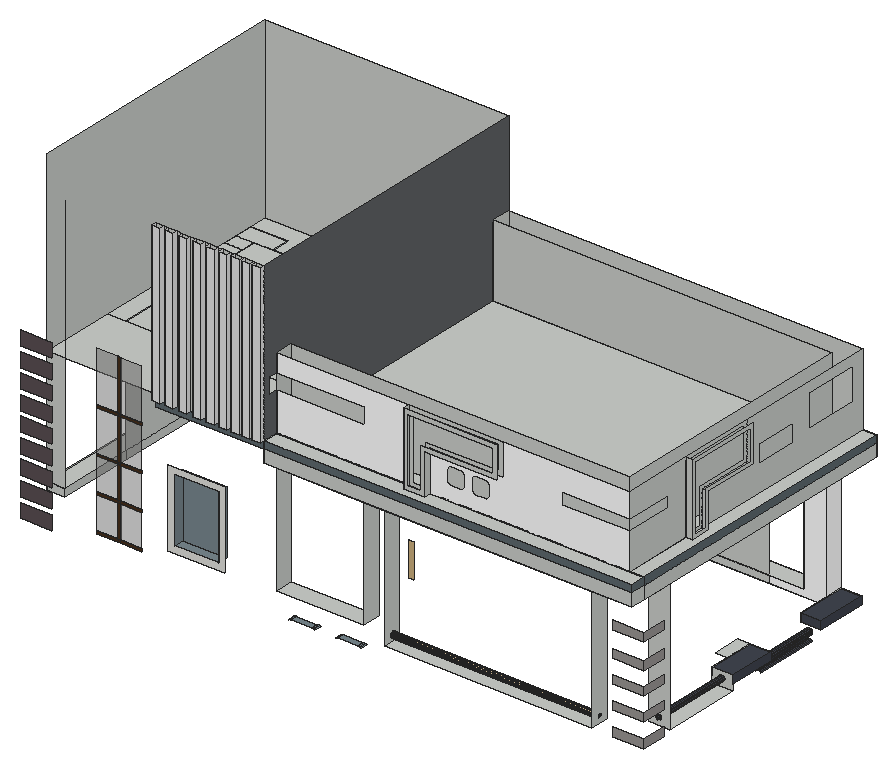
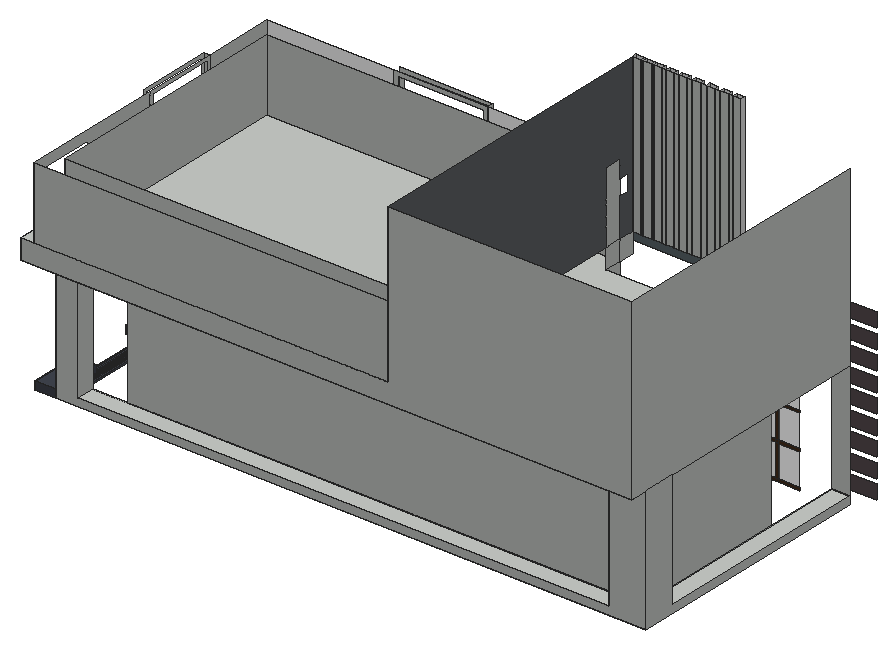
# SketchUp Ruby script. Lengths in inches.
U = 1.inch
M = Sketchup.active_model
def pt(a) = Geom::Point3d.new(a.map { |v| v * U })
def face(e, loops, mat)
  f = e.add_face(loops[0].map { |a| pt(a) })
  loops[1..].each { |l| e.add_face(l.map { |a| pt(a) }).erase! }
  f.material = f.back_material = mat if mat
  f
end
# faces: each face lists its corners as indices into pts; further lists are holes
def faces(e, pts, list, mat = nil) = list.each { |f| face(e, (f[0].is_a?(Array) ? f : [f]).map { |l| l.map { |i| pts[i] } }, mat) }
# xy, xz, yz: faces in a plane at the given z, y or x. An outline is a flat list of corners, or four numbers for a rectangle; further outlines are holes
def ring(l) = l.size == 4 ? [[l[0], l[1]], [l[2], l[1]], [l[2], l[3]], [l[0], l[3]]] : l.each_slice(2).to_a
def flat(e, list, mat, &to3) = list.each { |f| face(e, (f[0].is_a?(Array) ? f : [f]).map { |l| ring(l).map { |u, v| to3.(u, v) } }, mat) }
def xy(e, z, list, mat = nil) = flat(e, list, mat) { |x, y| [x, y, z] }
def xz(e, y, list, mat = nil) = flat(e, list, mat) { |x, z| [x, y, z] }
def yz(e, x, list, mat = nil) = flat(e, list, mat) { |y, z| [x, y, z] }
def lines(e, pts, list) = list.each { |a, b| e.add_line(pt(pts[a]), pt(pts[b])) }
# prism: a flat outline (further loops are holes) pulled along v
def prism(e, loops, v, mat = nil)
  f = face(e, loops, mat); d = Geom::Vector3d.new(v.map { |x| x * U })
  f.pushpull(f.normal.samedirection?(d) ? d.length : -d.length)
end
def box(e, o, s, mat = nil) = prism(e, [[o, [o[0] + s[0], o[1], o[2]], [o[0] + s[0], o[1] + s[1], o[2]], [o[0], o[1] + s[1], o[2]]]], [0, 0, s[2]], mat)
def at(x, y, z, deg = 0) = Geom::Transformation.translation(pt([x, y, z])) * Geom::Transformation.rotation(ORIGIN, Z_AXIS, deg.degrees)
def axes(o, x, y, z) = Geom::Transformation.new([*x, 0, *y, 0, *z, 0, *pt(o).to_a, 1])
def part(name) = M.definitions.add(name)
# library, detail: a bought-in or finely detailed component or shape, given as its bounding box
def library(name, o, s) = part(name).tap { |d| box(d.entities, o, s) }
def detail(e, o, s) = box(e.add_group.entities, o, s)
def put(e, d, t, mat = nil) = e.add_instance(d, t).tap { |i| i.material = mat if mat }
def group(e, t, mat = nil) = e.add_group.tap { |g| g.transformation = t; g.material = mat if mat }.entities
root = M.entities
M.materials.add("[Asphalt New]").color = [89, 79, 82]
M.materials.add("[Basic Tile]").color = [203, 206, 202]
M.materials.add("[Blacktop Old 01]").color = [96, 99, 102]
M.materials.add("[Color M00]").color = [255, 255, 255]
M.materials.add("[Concrete Aggregate Smoke]").color = [154, 150, 148]
M.materials.add("[Formica Beige]").color = [211, 187, 149]
M.materials.add("[Formica Laminate Dark]1").color = [65, 69, 79]
M.materials.add("[Formica Speckled Grey]").color = [120, 135, 142]
M.materials.add("[Formica Speckled Grey]1").color = [94, 105, 111]
M.materials.add("[Polished Concrete Old]").color = [229, 229, 229]
M.materials.add("[Translucent Glass Gray]").color = [128, 128, 128]
M.materials["[Translucent Glass Gray]"].alpha = 0.5
M.materials.add("[Wood Floor Light]").color = [204, 176, 127]
M.materials.add("[Wood Floor]").color = [71, 48, 28]
xy(root,488.49,[[753.6875,719.27,788.57,730.52],[837.19,719.27,870.38,730.52]],"[Formica Speckled Grey]")
xy(root,496.0625,[[909.08,730.52,1278.64,762.76]],"[Basic Tile]")
xy(root,499.9375,[[1333.54,788.47,1370.47,928.88]],"[Basic Tile]")
xy(root,510.75,[[282.77,762.76,282.77,1215.04,1333.54,1215.04,1333.54,1182.79,315.01,1182.79,315.01,762.76],[1333.54,1125.19,1370.47,1215.04]],"[Basic Tile]")
xy(root,517.3125,[[716.67,730.52,872.91,762.76]],"[Basic Tile]")
xy(root,524.8125,[[282.77,762.76,315.01,1157.24],[1311.73,963.8,1333.54,1012.73],[348.88,1182.79,1294.14,1215.04]],"[Basic Tile]")
xy(root,524.8125,[[1333.54,928.88,1370.47,1012.73],[1333.54,1125.19,1370.47,1215.04]],"[Formica Laminate Dark]1")
xy(root,544.32,[[557.73,703.09,635.17,720.91]],"[Formica Speckled Grey]")
xy(root,658.7,[[557.73,703.09,635.17,720.91]],"[Formica Speckled Grey]")
xy(root,732.375,[[716.67,703.09,872.91,730.52],[872.91,703.09,909.08,730.52],[909.08,703.09,1278.64,730.52],[1278.64,703.09,1370.47,730.52],[716.67,730.52,716.67,762.76,282.77,762.76,282.77,898.23,1370.47,898.23,1370.47,788.47,1333.54,788.47,1333.54,762.76,1278.64,762.76,1278.64,730.52,909.08,730.52,909.08,762.76,872.91,762.76,872.91,730.52],
  [872.91,730.52,909.08,762.76],[1278.64,730.52,1370.47,762.76],[1333.54,762.76,1370.47,788.47],[282.77,898.23,315.01,1157.24],[315.01,898.23,1230.77,1182.79],
  [1230.77,898.23,1230.77,1247.67,1294.14,1247.67,1294.14,1182.79,1370.47,1182.79,1370.47,898.23],[282.77,1157.24,315.01,1182.79],[282.77,1182.79,348.88,1215.04],[348.88,1182.79,348.88,1215.04,282.77,1215.04,282.77,1247.67,1230.77,1247.67,1230.77,1182.79],[1294.14,1182.79,1333.54,1215.04],
  [1333.54,1182.79,1370.47,1215.04],[1294.14,1215.04,1370.47,1247.67]],"[Basic Tile]")
xy(root,767.875,[[523.06,695.28,537.89,703.09],[545.87,695.28,560.71,703.09],[570.43,695.28,585.27,703.09],[595.93,695.28,610.77,703.09],[619.62,695.28,634.46,703.09],
  [642.37,695.28,657.21,703.09],[664.18,695.28,679.02,703.09],[683.01,695.28,697.85,703.09],[701.84,695.28,716.67,703.09],[716.67,703.09,1370.47,703.09,1370.47,730.52,989.93,730.52,989.93,718.33,952.31,718.33,952.31,730.52,716.67,730.52],
  [952.31,718.33,989.93,730.52],[716.67,730.52,716.67,762.76,1319.77,762.76,1319.77,1212.51,1345.67,1212.51,1345.67,730.52],[1345.67,730.52,1370.47,730.52,1370.47,1247.67,1345.67,1247.67,1345.67,891.02,1356.61,891.02,1356.61,855.93,1345.67,855.93],[716.67,762.76,1319.77,1212.51],[1345.67,855.93,1356.61,891.02],
  [716.67,1212.51,1345.67,1247.67]],"[Basic Tile]")
xz(root,695.28,[[523.06,767.875,537.89,1047.125],[545.87,767.875,560.71,1047.125],[570.43,767.875,585.27,1047.125],[595.93,767.875,610.77,1047.125],[619.62,767.875,634.46,1047.125],
  [642.37,767.875,657.21,1047.125],[664.18,767.875,679.02,1047.125],[683.01,767.875,697.85,1047.125],[701.84,767.875,716.67,1047.125]],"[Polished Concrete Old]")
xz(root,703.09,[[[546.1,532.7,646.79,670.32],[557.73,544.32,635.17,658.7]]])
xz(root,703.09,[[282.77,492.08,338.2,517.33],[282.77,526.39,338.2,551.64],[282.77,560.7,338.2,585.95],[282.77,595.02,338.2,620.27],[282.77,629.33,338.2,654.58],
  [282.77,663.64,338.2,688.89],[282.77,697.95,338.2,723.2],[282.77,732.27,338.2,757.52],[282.77,766.58,338.2,791.83]],"[Asphalt New]")
xz(root,703.09,[[716.67,732.375,1370.47,754.78],[523.06,767.875,537.89,1047.125],[537.89,767.875,545.87,1047.125],[545.87,767.875,560.71,1047.125],[560.71,767.875,570.43,1047.125],
  [570.43,767.875,585.27,1047.125],[585.27,767.875,595.93,1047.125],[595.93,767.875,610.77,1047.125],[610.77,767.875,619.62,1047.125],[619.62,767.875,634.46,1047.125],
  [634.46,767.875,642.37,1047.125],[642.37,767.875,657.21,1047.125],[657.21,767.875,664.18,1047.125],[664.18,767.875,679.02,1047.125],[679.02,767.875,683.01,1047.125],
  [683.01,767.875,697.85,1047.125],[697.85,767.875,701.84,1047.125],[701.84,767.875,716.67,1047.125]],"[Basic Tile]")
xz(root,703.09,[[523.06,754.78,716.67,767.875],[716.67,754.78,1370.47,767.875]],"[Formica Speckled Grey]1")
xz(root,718.33,[[[952.31,767.875,989.93,767.875,989.93,840.25,1118.75,840.25,1118.75,895.9375,952.31,895.9375],[958.95,774.51,958.95,889.3,1112.11,889.3,1112.11,846.89,983.3,846.89,983.3,774.51]]],"[Basic Tile]")
xz(root,720.91,[[557.73,544.32,635.17,658.7]],"[Formica Speckled Grey]")
xz(root,730.52,[[716.67,732.375,1370.47,767.875],[[952.31,767.875,952.31,895.9375,1118.75,895.9375,1118.75,840.25,989.93,840.25,989.93,767.875],[958.95,774.51,983.3,774.51,983.3,846.89,1112.11,846.89,1112.11,889.3,958.95,889.3]]],"[Basic Tile]")
xz(root,730.52,[[716.67,767.875,952.31,767.875,952.31,895.9375,716.67,895.9375,716.67,864.5625,873.36,864.5625,873.36,836.5625,716.67,836.5625],[[989.93,767.875,1345.67,767.875,1345.67,832.66,1224.56,832.66,1224.56,852.16,1345.67,852.16,1345.67,895.9375,1118.75,895.9375,1118.75,840.25,989.93,840.25],[1071.21,793.37,1070.34,793.43,1069.48,793.6,1068.65,793.88,1067.87,794.27,1067.14,794.75,1066.48,795.33,1065.9,795.99,1065.41,796.72,1065.03,797.5,1064.75,798.33,1064.57,799.19,1064.52,800.07,1064.52,817.85,1064.58,818.76,1064.75,819.65,1065.05,820.51,1065.45,821.33,1065.95,822.09,1066.55,822.77,1067.24,823.37,1067.99,823.875,1068.81,824.28,1069.67,824.57,1070.5625,824.75,1071.47,824.81,1088.97,824.81,1089.88,824.75,1090.78,824.57,1091.64,824.28,1092.46,823.87,1093.22,823.36,1093.91,822.76,1094.51,822.07,1095.02,821.31,1095.42,820.49,1095.72,819.63,1095.89,818.73,1095.95,817.82,1095.95,800.52,1095.89,799.59,1095.71,798.67,1095.41,797.79,1095,796.95,1094.48,796.17,1093.86,795.47,1093.16,794.85,1092.38,794.33,1091.54,793.91,1090.65,793.61,1089.74,793.43,1088.8,793.37],[1026.3,793.37,1025.49,793.42,1024.6875,793.58,1023.92,793.84,1023.1875,794.2,1022.51,794.66,1021.9,795.19,1021.36,795.8,1020.91,796.48,1020.55,797.21,1020.29,797.98,1020.13,798.78,1020.08,799.59,1020.08,814.88,1020.16,816.18,1020.42,817.45,1020.83,818.68,1021.41,819.84,1022.13,820.92,1022.99,821.9,1023.96,822.76,1025.04,823.48,1026.21,824.05,1027.4375,824.47,1028.71,824.72,1030.01,824.81,1043.7,824.81,1044.72,824.74,1045.72,824.54,1046.6875,824.21,1047.61,823.76,1048.46,823.19,1049.23,822.52,1049.9,821.75,1050.47,820.9,1050.92,819.98,1051.25,819.01,1051.45,818.01,1051.52,816.99,1051.52,799.87,1051.46,799.02,1051.3,798.19,1051.02,797.38,1050.65,796.62,1050.17,795.91,1049.61,795.27,1048.98,794.71,1048.27,794.24,1047.51,793.86,1046.7,793.59,1045.87,793.43,1045.02,793.37]]],"[Color M00]")
xz(root,730.52,[[1314.99,494.79,1370.47,509.54],[1314.99,536.91,1370.47,551.66],[1314.99,578.29,1370.47,593.04],[1314.99,619.47,1370.47,634.22],[1314.99,665.22,1370.47,679.97]],"[Concrete Aggregate Smoke]")
xz(root,741.66,[[387.85,492.35,425.21,549.53],[430.65,492.35,468.81,549.53],[387.85,554.52,425.21,611.26],[430.65,554.52,468.81,611.26],[387.85,615.28,425.21,688.12],
  [430.65,615.28,468.81,688.12],[387.85,692.61,425.21,783.4],[430.65,692.61,468.81,783.4]],"[Translucent Glass Gray]")
xz(root,741.66,[[387.85,487.63,425.21,492.35],[425.21,487.63,430.65,492.35],[430.65,487.63,468.81,492.35],[425.21,492.35,430.65,549.53],[387.85,549.53,425.21,554.52],
  [425.21,549.53,430.65,554.52],[430.65,549.53,468.81,554.52],[425.21,554.52,430.65,611.26],[387.85,611.26,425.21,615.28],[425.21,611.26,430.65,615.28],
  [430.65,611.26,468.81,615.28],[425.21,615.28,430.65,688.12],[387.85,688.12,425.21,692.61],[425.21,688.12,430.65,692.61],[430.65,688.12,468.81,692.61],
  [425.21,692.61,430.65,783.4]],"[Wood Floor]")
xz(root,762.76,[[282.77,510.75,315.01,524.8125],[282.77,524.8125,315.01,732.375],[716.67,767.875,1319.77,895.9375]],"[Basic Tile]")
xz(root,788.47,[[[1333.54,499.9375,1370.47,732.375],[1350.59,508.02,1351.82,508.18,1352.97,508.66,1353.95,509.41,1354.71,510.4,1355.18,511.54,1355.34,512.77,1355.18,514,1354.71,515.15,1353.95,516.13,1352.97,516.89,1351.82,517.36,1350.59,517.52,1349.37,517.36,1348.22,516.89,1347.24,516.13,1346.48,515.15,1346.01,514,1345.84,512.77,1346.01,511.54,1346.48,510.4,1347.24,509.41,1348.22,508.66,1349.37,508.18]]],"[Basic Tile]")
xz(root,855.93,[[1345.67,767.875,1356.61,895.9375]],"[Basic Tile]")
xz(root,891.02,[[1345.67,767.875,1356.61,829.875]],"[Basic Tile]")
xz(root,898.23,[[817.84,499.54,826.9,559.11]],"[Wood Floor Light]")
xz(root,928.88,[[[1333.54,499.9375,1370.47,524.8125],[1350.59,508.02,1349.37,508.18,1348.22,508.66,1347.24,509.41,1346.48,510.4,1346.01,511.54,1345.84,512.77,1346.01,514,1346.48,515.15,1347.24,516.13,1348.22,516.89,1349.37,517.36,1350.59,517.52,1351.82,517.36,1352.97,516.89,1353.95,516.13,1354.71,515.15,1355.18,514,1355.34,512.77,1355.18,511.54,1354.71,510.4,1353.95,509.41,1352.97,508.66,1351.82,508.18]],[1350.59,508.02,1349.37,508.18,1348.22,508.66,1347.24,509.41,1346.48,510.4,1346.01,511.54,1345.84,512.77,1346.01,514,1346.48,515.15,1347.24,516.13,1348.22,516.89,1349.37,517.36,1350.59,517.52,1351.82,517.36,1352.97,516.89,1353.95,516.13,1354.71,515.15,1355.18,514,1355.34,512.77,1355.18,511.54,1354.71,510.4,1353.95,509.41,1352.97,508.66,1351.82,508.18]],"[Basic Tile]")
xz(root,1012.73,[[1333.54,510.75,1370.47,524.8125]],"[Formica Laminate Dark]1")
xz(root,1125.19,[[1349.2,495.79,1347.875,495.97,1346.64,496.48,1345.58,497.29,1344.76,498.35,1344.25,499.59,1344.08,500.92,1344.25,502.24,1344.76,503.48,1345.58,504.54,1346.64,505.36,1347.875,505.87,1349.2,506.04,1350.53,505.87,1351.77,505.36,1352.83,504.54,1353.64,503.48,1354.15,502.24,1354.33,500.92,1354.15,499.59,1353.64,498.35,1352.83,497.29,1351.77,496.48,1350.53,495.97]],"[Basic Tile]")
xz(root,1125.19,[[1333.54,510.75,1370.47,524.8125]],"[Formica Laminate Dark]1")
xz(root,1157.24,[[282.77,524.8125,315.01,732.375]],"[Basic Tile]")
xz(root,1182.79,[[315.01,510.75,315.01,732.375,348.88,732.375,348.88,524.8125,1230.77,524.8125,1230.77,510.75],[348.88,524.8125,1230.77,732.375]],"[Basic Tile]")
xz(root,1182.79,[[1230.77,510.75,1333.54,510.75,1333.54,732.375,1294.14,732.375,1294.14,524.8125,1230.77,524.8125]],"[Color M00]")
xz(root,1212.51,[[716.67,767.875,1319.77,895.9375]],"[Basic Tile]")
xz(root,1215.04,[[282.77,510.75,282.77,732.375,348.88,732.375,348.88,524.8125,1294.14,524.8125,1294.14,732.375,1333.54,732.375,1333.54,510.75]],"[Basic Tile]")
xz(root,1215.04,[[1333.54,510.75,1370.47,524.8125]],"[Formica Laminate Dark]1")
xz(root,1247.67,[[282.77,732.375,282.77,1047.125,716.67,1047.125,716.67,767.875,1370.47,767.875,1370.47,732.375],[716.67,767.875,1345.67,895.9375]],"[Basic Tile]")
yz(root,282.77,[[762.76,510.75,762.76,524.8125,1157.24,524.8125,1157.24,732.375,1215.04,732.375,1215.04,510.75],[762.76,732.375,1247.67,1047.125]],"[Basic Tile]")
yz(root,315.01,[[762.76,510.75,898.23,524.8125],[898.23,510.75,898.23,524.8125,1157.24,524.8125,1157.24,732.375,1182.79,732.375,1182.79,510.75],[898.23,524.8125,1157.24,732.375]],"[Basic Tile]")
yz(root,348.88,[[1182.79,524.8125,1215.04,732.375]],"[Basic Tile]")
yz(root,523.06,[[695.28,767.875,703.09,1047.125]],"[Polished Concrete Old]")
yz(root,537.89,[[695.28,767.875,703.09,1047.125]],"[Polished Concrete Old]")
yz(root,545.87,[[695.28,767.875,703.09,1047.125]],"[Polished Concrete Old]")
yz(root,557.73,[[703.09,544.32,720.91,658.7]],"[Formica Speckled Grey]")
yz(root,560.71,[[695.28,767.875,703.09,1047.125]],"[Polished Concrete Old]")
yz(root,570.43,[[695.28,767.875,703.09,1047.125]],"[Polished Concrete Old]")
yz(root,585.27,[[695.28,767.875,703.09,1047.125]],"[Polished Concrete Old]")
yz(root,595.93,[[695.28,767.875,703.09,1047.125]],"[Polished Concrete Old]")
yz(root,610.77,[[695.28,767.875,703.09,1047.125]],"[Polished Concrete Old]")
yz(root,619.62,[[695.28,767.875,703.09,1047.125]],"[Polished Concrete Old]")
yz(root,634.46,[[695.28,767.875,703.09,1047.125]],"[Polished Concrete Old]")
yz(root,635.17,[[703.09,544.32,720.91,658.7]],"[Formica Speckled Grey]")
yz(root,642.37,[[695.28,767.875,703.09,1047.125]],"[Polished Concrete Old]")
yz(root,657.21,[[695.28,767.875,703.09,1047.125]],"[Polished Concrete Old]")
yz(root,664.18,[[695.28,767.875,703.09,1047.125]],"[Polished Concrete Old]")
yz(root,679.02,[[695.28,767.875,703.09,1047.125]],"[Polished Concrete Old]")
yz(root,683.01,[[695.28,767.875,703.09,1047.125]],"[Polished Concrete Old]")
yz(root,697.85,[[695.28,767.875,703.09,1047.125]],"[Polished Concrete Old]")
yz(root,701.84,[[695.28,767.875,703.09,1047.125]],"[Polished Concrete Old]")
yz(root,716.67,[[730.52,517.3125,762.76,732.375],[703.09,732.375,730.52,767.875],[730.52,732.375,762.76,767.875],[730.52,767.875,762.76,895.9375],[1212.51,767.875,1247.67,895.9375]],"[Basic Tile]")
yz(root,716.67,[[703.09,767.875,730.52,767.875,730.52,836.5625,713.41,836.5625,713.41,864.5625,730.52,864.5625,730.52,895.9375,762.76,895.9375,762.76,767.875,1212.51,767.875,1212.51,895.9375,1247.67,895.9375,1247.67,1047.125,703.09,1047.125]],"[Blacktop Old 01]")
yz(root,716.67,[[695.28,767.875,703.09,1047.125]],"[Polished Concrete Old]")
yz(root,872.91,[[730.52,517.3125,762.76,732.375]],"[Basic Tile]")
yz(root,909.08,[[[730.52,496.0625,762.76,732.375],[747.21,502.82,745.98,502.98,744.84,503.45,743.85,504.21,743.1,505.19,742.625,506.34,742.46,507.57,742.625,508.8,743.1,509.94,743.85,510.93,744.84,511.68,745.98,512.15,747.21,512.32,748.44,512.15,749.59,511.68,750.57,510.93,751.33,509.94,751.8,508.8,751.96,507.57,751.8,506.34,751.33,505.19,750.57,504.21,749.59,503.45,748.44,502.98]],[747.21,502.82,745.98,502.98,744.84,503.45,743.85,504.21,743.1,505.19,742.625,506.34,742.46,507.57,742.625,508.8,743.1,509.94,743.85,510.93,744.84,511.68,745.98,512.15,747.21,512.32,748.44,512.15,749.59,511.68,750.57,510.93,751.33,509.94,751.8,508.8,751.96,507.57,751.8,506.34,751.33,505.19,750.57,504.21,749.59,503.45,748.44,502.98]],"[Basic Tile]")
yz(root,952.31,[[718.33,767.875,730.52,895.9375]],"[Basic Tile]")
yz(root,989.93,[[718.33,767.875,730.52,840.25]],"[Basic Tile]")
yz(root,1278.64,[[[730.52,496.0625,762.76,732.375],[747.21,502.82,748.44,502.98,749.59,503.45,750.57,504.21,751.33,505.19,751.8,506.34,751.96,507.57,751.8,508.8,751.33,509.94,750.57,510.93,749.59,511.68,748.44,512.15,747.21,512.32,745.98,512.15,744.84,511.68,743.85,510.93,743.1,509.94,742.625,508.8,742.46,507.57,742.625,506.34,743.1,505.19,743.85,504.21,744.84,503.45,745.98,502.98]]],"[Basic Tile]")
yz(root,1294.14,[[1182.79,524.8125,1215.04,732.375]],"[Basic Tile]")
yz(root,1319.77,[[762.76,767.875,1212.51,895.9375]],"[Basic Tile]")
yz(root,1333.54,[[928.88,510.75,963.8,524.8125],[963.8,510.75,1012.73,524.8125],[1182.79,510.75,1215.04,524.8125]],"[Basic Tile]")
yz(root,1333.54,[[1182.79,524.8125,1215.04,732.375]],"[Color M00]")
yz(root,1333.54,[[1125.19,510.75,1182.79,524.8125]],"[Formica Laminate Dark]1")
yz(root,1345.67,[[730.52,767.875,855.93,767.875,855.93,895.9375,730.52,895.9375,730.52,852.16,814.64,852.16,814.64,832.66,730.52,832.66],[[855.93,767.875,855.93,895.9375,990.33,895.9375,990.33,829.875,891.02,829.875,891.02,767.875],[861.53,773.48,885.41,773.48,885.41,835.48,984.72,835.48,984.72,890.33,861.53,890.33]],[[891.02,767.875,1247.67,767.875,1247.67,895.9375,990.33,895.9375,990.33,829.875,891.02,829.875],[1128.05,821.08,1226.23,878.58],[1016.59,814.05,1093.89,846.55]]],"[Basic Tile]")
yz(root,1356.61,[[[855.93,767.875,891.02,767.875,891.02,829.875,990.33,829.875,990.33,895.9375,855.93,895.9375],[861.53,773.48,861.53,890.33,984.72,890.33,984.72,835.48,885.41,835.48,885.41,773.48]]],"[Basic Tile]")
yz(root,1370.47,[[703.09,732.375,730.52,754.78],[730.52,732.375,1247.67,754.78]],"[Basic Tile]")
yz(root,1370.47,[[730.52,494.79,774.21,509.54],[730.52,536.91,774.21,551.66],[730.52,578.29,774.21,593.04],[730.52,619.47,774.21,634.22],[730.52,665.22,774.21,679.97]],"[Concrete Aggregate Smoke]")
yz(root,1370.47,[[928.88,510.75,1012.73,524.8125],[1125.19,510.75,1215.04,524.8125]],"[Formica Laminate Dark]1")
yz(root,1370.47,[[703.09,754.78,730.52,767.875],[730.52,754.78,1247.67,767.875]],"[Formica Speckled Grey]1")
p = [[1345.58,1125.19,487.54],[1344.76,1125.19,486.48],[1344.76,1012.73,486.48],[1345.58,1012.73,487.54],[1353.64,1125.19,486.48],[1352.83,1125.19,487.54],
  [1352.83,1012.73,487.54],[1353.64,1012.73,486.48],[877.55,730.52,486.57],[875.87,730.52,487.4],[875.87,719.27,487.4],[877.55,719.27,486.57],
  [748.87,730.52,487.53],[747.39,730.52,486.8],[747.39,719.27,486.8],[748.87,719.27,487.53],[794.77,730.52,486.83],[793.32,730.52,487.55],
  [793.32,719.27,487.55],[794.77,719.27,486.83],[832.46,730.52,487.55],[831.02,730.52,486.84],[831.02,719.27,486.84],[832.46,719.27,487.55],
  [874.09,730.52,488],[874.09,719.27,488],[750.43,730.52,488.0625],[750.43,719.27,488.0625],[791.78,730.52,488.07],[791.78,719.27,488.07],
  [1346.64,1125.19,488.36],[1346.64,1012.73,488.36],[1351.77,1125.19,488.36],[1351.77,1012.73,488.36],[833.99,730.52,488.07],[833.99,719.27,488.07],
  [872.25,730.52,488.37],[872.25,719.27,488.37],[752.04,730.52,488.38],[752.04,719.27,488.38],[790.19,730.52,488.39],[790.19,719.27,488.39],
  [835.58,730.52,488.39],[835.58,719.27,488.39],[753.6875,730.52,488.49],[753.6875,719.27,488.49],[788.57,730.52,488.49],[788.57,719.27,488.49],
  [837.19,730.52,488.49],[837.19,719.27,488.49],[870.38,730.52,488.49],[870.38,719.27,488.49],[1347.875,1125.19,488.87],[1347.875,1012.73,488.87],
  [1350.53,1125.19,488.87],[1350.53,1012.73,488.87],[1349.2,1125.19,489.04],[1349.2,1012.73,489.04],[1347.875,1125.19,495.97],[1349.2,1125.19,495.79],
  [1349.2,1012.73,495.79],[1347.875,1012.73,495.97],[1350.53,1125.19,495.97],[1350.53,1012.73,495.97],[1346.64,1125.19,496.48],[1346.64,1012.73,496.48],
  [1351.77,1125.19,496.48],[1351.77,1012.73,496.48],[1345.58,1125.19,497.29],[1345.58,1012.73,497.29],[1352.83,1125.19,497.29],[1352.83,1012.73,497.29],
  [1344.76,1125.19,498.35],[1344.76,1012.73,498.35],[1353.64,1125.19,498.35],[1353.64,1012.73,498.35],[1344.25,1125.19,499.59],[1344.25,1012.73,499.59],
  [1354.15,1125.19,499.59],[1354.15,1012.73,499.59],[1344.08,1125.19,500.92],[1344.08,1012.73,500.92],[1354.33,1125.19,500.92],[1354.33,1012.73,500.92],
  [1344.25,1125.19,502.24],[1344.25,1012.73,502.24],[1354.15,1125.19,502.24],[1354.15,1012.73,502.24],[1344.76,1125.19,503.48],[1344.76,1012.73,503.48],
  [1353.64,1125.19,503.48],[1353.64,1012.73,503.48],[909.08,745.98,502.98],[909.08,747.21,502.82],[1278.64,747.21,502.82],[1278.64,745.98,502.98],
  [909.08,748.44,502.98],[1278.64,748.44,502.98],[909.08,744.84,503.45],[1278.64,744.84,503.45],[909.08,749.59,503.45],[1278.64,749.59,503.45],
  [909.08,743.85,504.21],[1278.64,743.85,504.21],[909.08,750.57,504.21],[1278.64,750.57,504.21],[1345.58,1125.19,504.54],[1345.58,1012.73,504.54],
  [1352.83,1125.19,504.54],[1352.83,1012.73,504.54],[909.08,743.1,505.19],[1278.64,743.1,505.19],[909.08,751.33,505.19],[1278.64,751.33,505.19],
  [1346.64,1125.19,505.36],[1346.64,1012.73,505.36],[1351.77,1125.19,505.36],[1351.77,1012.73,505.36],[909.08,742.625,506.34],[1278.64,742.625,506.34],
  [909.08,751.8,506.34],[1278.64,751.8,506.34],[1347.875,1125.19,505.87],[1347.875,1012.73,505.87],[1350.53,1125.19,505.87],[1350.53,1012.73,505.87],
  [1349.2,1125.19,506.04],[1349.2,1012.73,506.04],[909.08,742.46,507.57],[1278.64,742.46,507.57],[909.08,751.96,507.57],[1278.64,751.96,507.57],
  [909.08,742.625,508.8],[1278.64,742.625,508.8],[909.08,751.8,508.8],[1278.64,751.8,508.8],[1349.37,928.88,508.18],[1350.59,928.88,508.02],
  [1350.59,788.47,508.02],[1349.37,788.47,508.18],[1351.82,928.88,508.18],[1351.82,788.47,508.18],[1348.22,928.88,508.66],[1348.22,788.47,508.66],
  [1352.97,928.88,508.66],[1352.97,788.47,508.66],[1347.24,928.88,509.41],[1347.24,788.47,509.41],[1353.95,928.88,509.41],[1353.95,788.47,509.41],
  [909.08,743.1,509.94],[1278.64,743.1,509.94],[909.08,751.33,509.94],[1278.64,751.33,509.94],[1346.48,928.88,510.4],[1346.48,788.47,510.4],
  [1354.71,928.88,510.4],[1354.71,788.47,510.4],[909.08,743.85,510.93],[1278.64,743.85,510.93],[909.08,750.57,510.93],[1278.64,750.57,510.93],
  [1346.01,928.88,511.54],[1346.01,788.47,511.54],[1355.18,928.88,511.54],[1355.18,788.47,511.54],[909.08,744.84,511.68],[1278.64,744.84,511.68],
  [909.08,749.59,511.68],[1278.64,749.59,511.68],[1345.84,928.88,512.77],[1345.84,788.47,512.77],[1355.34,928.88,512.77],[1355.34,788.47,512.77],
  [909.08,745.98,512.15],[1278.64,745.98,512.15],[909.08,748.44,512.15],[1278.64,748.44,512.15],[909.08,747.21,512.32],[1278.64,747.21,512.32],
  [1346.01,928.88,514],[1346.01,788.47,514],[1355.18,928.88,514],[1355.18,788.47,514],[1346.48,928.88,515.15],[1346.48,788.47,515.15],
  [1354.71,928.88,515.15],[1354.71,788.47,515.15],[1347.24,928.88,516.13],[1347.24,788.47,516.13],[1353.95,928.88,516.13],[1353.95,788.47,516.13],
  [1348.22,928.88,516.89],[1348.22,788.47,516.89],[1352.97,928.88,516.89],[1352.97,788.47,516.89],[1349.37,928.88,517.36],[1349.37,788.47,517.36],
  [1351.82,928.88,517.36],[1351.82,788.47,517.36],[1350.59,928.88,517.52],[1350.59,788.47,517.52],[315.01,762.76,732.375],[315.01,762.76,984.4375]]
faces(root,p,[[0,1,2,3],[4,5,6,7],[30,0,3,31],[5,32,33,6],[52,30,31,53],[32,54,55,33],[56,52,53,57],[54,56,57,55],
  [58,59,60,61],[59,62,63,60],[64,58,61,65],[62,66,67,63],[68,64,65,69],[66,70,71,67],[72,68,69,73],[70,74,75,71],
  [76,72,73,77],[74,78,79,75],[80,76,77,81],[78,82,83,79],[84,80,81,85],[82,86,87,83],[88,84,85,89],[86,90,91,87],
  [106,88,89,107],[90,108,109,91],[114,106,107,115],[108,116,117,109],[122,114,115,123],[116,124,125,117],[126,122,123,127],[124,126,127,125],
  [136,137,138,139],[137,140,141,138],[142,136,139,143],[140,144,145,141],[146,142,143,147],[144,148,149,145],[154,146,147,155],[148,156,157,149],
  [162,154,155,163],[156,164,165,157],[170,162,163,171],[164,172,173,165],[180,170,171,181],[172,182,183,173],[184,180,181,185],[182,186,187,183],
  [188,184,185,189],[186,190,191,187],[192,188,189,193],[190,194,195,191],[196,192,193,197],[194,198,199,195],[200,196,197,201],[198,200,201,199]],"[Formica Laminate Dark]1")
faces(root,p,[[8,9,10,11],[12,13,14,15],[16,17,18,19],[20,21,22,23],[9,24,25,10],[26,12,15,27],[17,28,29,18],[34,20,23,35],
  [24,36,37,25],[38,26,27,39],[28,40,41,29],[42,34,35,43],[44,38,39,45],[40,46,47,41],[48,42,43,49],[36,50,51,37]],"[Formica Speckled Grey]")
faces(root,p,[[92,93,94,95],[93,96,97,94],[98,92,95,99],[96,100,101,97],[102,98,99,103],[100,104,105,101],[110,102,103,111],[104,112,113,105],
  [118,110,111,119],[112,120,121,113],[128,118,119,129],[120,130,131,121],[132,128,129,133],[130,134,135,131],[150,132,133,151],[134,152,153,135],
  [158,150,151,159],[152,160,161,153],[166,158,159,167],[160,168,169,161],[174,166,167,175],[168,176,177,169],[178,174,175,179],[176,178,179,177]],"[Formica Beige]")
lines(root,p,[[202,203]])
